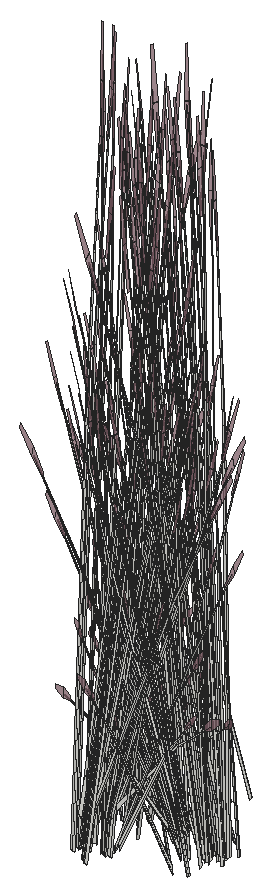
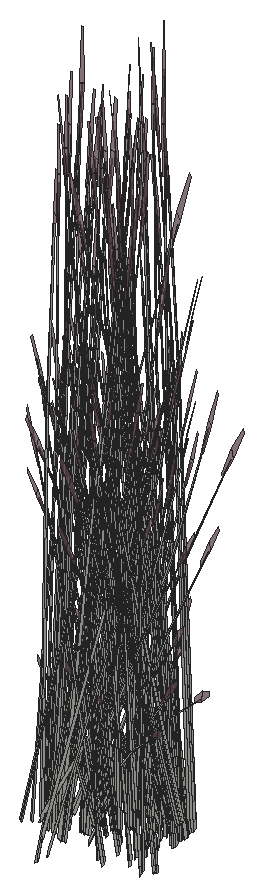
# SketchUp Ruby script. Lengths in inches.
U = 1.inch
M = Sketchup.active_model
def pt(a) = Geom::Point3d.new(a.map { |v| v * U })
def face(e, loops, mat)
  f = e.add_face(loops[0].map { |a| pt(a) })
  loops[1..].each { |l| e.add_face(l.map { |a| pt(a) }).erase! }
  f.material = f.back_material = mat if mat
  f
end
# faces: each face lists its corners as indices into pts; further lists are holes
def faces(e, pts, list, mat = nil) = list.each { |f| face(e, (f[0].is_a?(Array) ? f : [f]).map { |l| l.map { |i| pts[i] } }, mat) }
# xy, xz, yz: faces in a plane at the given z, y or x. An outline is a flat list of corners, or four numbers for a rectangle; further outlines are holes
def ring(l) = l.size == 4 ? [[l[0], l[1]], [l[2], l[1]], [l[2], l[3]], [l[0], l[3]]] : l.each_slice(2).to_a
def flat(e, list, mat, &to3) = list.each { |f| face(e, (f[0].is_a?(Array) ? f : [f]).map { |l| ring(l).map { |u, v| to3.(u, v) } }, mat) }
def xy(e, z, list, mat = nil) = flat(e, list, mat) { |x, y| [x, y, z] }
def xz(e, y, list, mat = nil) = flat(e, list, mat) { |x, z| [x, y, z] }
def yz(e, x, list, mat = nil) = flat(e, list, mat) { |y, z| [x, y, z] }
def lines(e, pts, list) = list.each { |a, b| e.add_line(pt(pts[a]), pt(pts[b])) }
# prism: a flat outline (further loops are holes) pulled along v
def prism(e, loops, v, mat = nil)
  f = face(e, loops, mat); d = Geom::Vector3d.new(v.map { |x| x * U })
  f.pushpull(f.normal.samedirection?(d) ? d.length : -d.length)
end
def box(e, o, s, mat = nil) = prism(e, [[o, [o[0] + s[0], o[1], o[2]], [o[0] + s[0], o[1] + s[1], o[2]], [o[0], o[1] + s[1], o[2]]]], [0, 0, s[2]], mat)
def at(x, y, z, deg = 0) = Geom::Transformation.translation(pt([x, y, z])) * Geom::Transformation.rotation(ORIGIN, Z_AXIS, deg.degrees)
def axes(o, x, y, z) = Geom::Transformation.new([*x, 0, *y, 0, *z, 0, *pt(o).to_a, 1])
def part(name) = M.definitions.add(name)
# library, detail: a bought-in or finely detailed component or shape, given as its bounding box
def library(name, o, s) = part(name).tap { |d| box(d.entities, o, s) }
def detail(e, o, s) = box(e.add_group.entities, o, s)
def put(e, d, t, mat = nil) = e.add_instance(d, t).tap { |i| i.material = mat if mat }
def group(e, t, mat = nil) = e.add_group.tap { |g| g.transformation = t; g.material = mat if mat }.entities
root = M.entities
M.materials.add("LightPink_Translucent").color = [144, 107, 117]
M.materials["LightPink_Translucent"].alpha = 0.75
c1 = part("blade")
p = [[2.15,0.21,22],[0,0.17,0],[0.09,0.45,0],[2.18,0.31,22],[2.29,0.31,22],[0.38,0.45,0],
  [2.48,0.24,33],[2.49,0.24,33],[2.48,0.22,33]]
faces(c1.entities,p,[[0,1,2,3],[4,5,2,3],[6,3,4,7],[8,0,3,6]])
c2 = part("seeds")
p = [[0.3,-0.1,1.38],[-0.01,-0.03,1.59],[-0.01,-0.03,0.03],[0.14,-0.07,-0.07],[0.29,-0.03,3],[0.15,0.01,3.11]]
faces(c2.entities,p,[[0,1,2,3],[1,0,4,5]],"LightPink_Translucent")
c3 = part("blade with seeds")
put(c3.entities,c1,at(0,0,0))
put(c3.entities,c2,axes([2.4,0.25,30.99],[1.5799,-0.05474,1.17369],[-0.12525,1.92788,0.29478],[-0.07173,-0.02425,1.56792]))
put(root,c3,axes([315.02,25.22,44.4],[-0.30332,-0.32798,0.39531],[0.45944,-0.23096,-0.19025],[0.09816,0.04058,1.26923]))
put(root,c3,axes([315.18,25.25,44.36],[0.50979,-0.25942,-0.25709],[0.339,0.36656,-0.44182],[0.12578,0.03723,1.41118]))
put(root,c3,axes([317.2,25.93,46],[0.41962,0.10901,-0.31292],[-0.12239,0.31802,0.40398],[0.16894,-0.02916,0.77298]))
put(root,c3,axes([321.92,27.46,46.18],[0.22948,-0.24822,0.05682],[0.32679,0.14452,0.44729],[-0.10565,-0.07958,0.68204]))
put(root,c3,axes([321.03,27.43,43.32],[-0.04891,0.05148,1.55816],[-0.49427,0.11098,-0.23804],[-0.1194,-0.10096,0.26541]))
put(root,c3,axes([316.46,24.56,43.78],[0.47255,0.19538,-0.43871],[-0.28245,0.35034,0],[0.10763,0.0445,1.3917]))
put(root,c3,axes([315.5625,25.67,43.95],[0.56491,0,0],[0,0.40454,0],[0,0,1.5764]))
put(root,c3,axes([321.85,28.84,43.85],[-0.20736,-0.4007,-0.61707],[0.59731,-0.14431,-0.16195],[-0.02292,-0.13569,1.36206]))
put(root,c3,axes([320.77,27.95,45.43],[0.18755,0.06732,1.51428],[-0.38813,0.28243,0.12244],[-0.24191,-0.12741,0.64734]))
put(root,c3,axes([315.72,24.72,44.1875],[-0.54257,0.10371,0.15589],[-0.13397,-0.38597,0.31002],[0.04839,0.05624,1.41735]))
put(root,c3,axes([316.06,25.54,45.43],[-0.20943,0.00885,1.51428],[0.13893,-0.38357,0.12244],[0.29846,0.02372,0.64734]))
put(root,c3,axes([323.06,27.7,46.46],[-0.15222,0.30049,0.31292],[-0.44409,-0.08764,-0.40398],[-0.04072,-0.12098,0.77298]))
put(root,c3,axes([316.33,24.7,43.79],[0.11861,0.34048,-0.27372],[-0.47106,0.09668,0.27372],[0.09497,0.03926,1.22797]))
put(root,c3,axes([321.67,27.75,46.14],[-0.49824,0.09289,-0.45151],[-0.08716,-0.35177,-0.34973],[-0.13382,-0.10081,0.86392]))
put(root,c3,axes([317.14,26.0625,46.18],[0.18545,0.26643,0.05682],[-0.33817,0.13041,0.44729],[0.14907,-0.02573,0.68204]))
put(root,c3,axes([322.02,27.43,46.8],[-0.33698,0.3746,-0.12034],[-0.48801,-0.21581,-0.66795],[-0.16964,-0.10584,1.01494]))
put(root,c3,axes([315.38,25.46,44.1],[-0.63817,-0.08233,0.43472],[0.12987,-0.46497,0.17059],[0.09326,0.0449,1.50931]))
put(root,c3,axes([317.11,25.97,46.18],[-0.14265,0.35629,0.42415],[-0.46898,-0.12183,0.34973],[0.18443,-0.02141,0.87768]))
put(root,c3,axes([315.49,26.57,43.93],[0.53009,-0.13258,-0.16963],[0.18627,0.38191,0.00007],[0.05851,-0.01465,1.53656]))
put(root,c3,axes([322.46,27.22,43.88],[-0.34892,0.22417,-0.0344],[-0.3197,-0.24551,-0.15595],[-0.02251,-0.06957,0.51438]))
put(root,c3,axes([315.55,25.84,43.96],[0.35245,0.2524,0],[-0.35245,0.2524,0],[0,0,1.49564]))
put(root,c3,axes([315.77,25.3,43.82],[0.52523,0.06406,-0.55095],[-0.11084,0.39517,-0.1446],[0.15674,0.04788,1.21613]))
put(root,c3,axes([320.73,27.33,46.17],[-0.10864,-0.00276,1.54581],[-0.34587,0.27582,-0.24447],[-0.18454,-0.05636,0.12397]))
put(root,c3,axes([318.09,25.99,44.44],[-0.31197,0.06451,1.01491],[0.14684,-0.26661,0.74569],[0.1655,0.01824,0.22354]))
put(root,c3,axes([315.6875,29.41,44.29],[-0.14352,0.07909,1.26356],[-0.42983,-0.13843,-0.27174],[0.07968,-0.17216,0.54024]))
put(root,c3,axes([322.91,29.875,44.9375],[0.43633,0.15757,1.33654],[-0.42745,0.33945,0.52853],[-0.19146,-0.20119,1.12046]))
put(root,c3,axes([315.55,25.55,44.4],[0.24498,-0.3521,0.39531],[0.50902,0.16945,-0.19025],[0,0.08116,1.26923]))
put(root,c3,axes([317.95,27.12,46.16],[-0.04566,-0.03421,1.56736],[0.09987,-0.36669,-0.1481],[0.17984,-0.02343,0.27737]))
put(root,c3,axes([321.99,27.75,46.46],[0.07798,0.31474,0.31292],[-0.44579,0.08311,-0.40398],[-0.11974,-0.09019,0.77298]))
put(root,c3,axes([320.625,28.79,43.78],[0,-0.39075,-0.43871],[0.56491,0,0],[0,-0.089,1.3917]))
put(root,c3,axes([320.65,27.95,46.5],[0.41698,-0.28837,0.47505],[0.35962,0.30624,0.3917],[-0.19563,-0.05319,0.983]))
put(root,c3,axes([315.5,25.43,43.95],[0.30332,0.32798,-0.39531],[-0.45944,0.23096,0.19025],[0.09816,0.04058,1.26923]))
put(root,c3,axes([317.55,26.82,45.47],[-0.09664,-0.32847,-0.03085],[0.45676,-0.07551,-0.13989],[0.09538,0.02082,0.4614]))
put(root,c3,axes([316.04,29.99,46.4],[0.01314,-0.36145,-0.62776],[0.55324,0.02428,0.07576],[0.05838,-0.15313,0.88802]))
put(root,c3,axes([316.37,26.81,46.45],[0.02704,-0.39739,-0.10745],[0.51189,0.01086,-0.59638],[0.19715,0.0276,0.90619]))
put(root,c3,axes([316.83,25.75,44.19],[0,-0.39075,0.43871],[0.56491,0,0],[0,0.089,1.3917]))
put(root,c3,axes([316.81,29.43,46.17],[-0.00487,-0.07777,1.54581],[-0.41166,-0.22476,-0.24447],[0.06364,-0.13625,0.12397]))
put(root,c3,axes([315.41,29.8125,45.43],[-0.09401,0.13431,1.51428],[-0.3944,-0.27795,0.12244],[0.17792,-0.17323,0.64734]))
put(root,c3,axes([316.7,29.15,46.16],[-0.05128,0.02985,1.56736],[-0.5024,-0.1007,-0.1481],[-0.01819,-0.13025,0.27737]))
put(root,c3,axes([315.76,25.63,44.3125],[0.47043,-0.11396,0.12794],[0.16474,0.32541,-0.36534],[0,0.07162,1.11991]))
put(root,c3,axes([316.29,26.65,46.46],[-0.28729,-0.24465,0.31292],[0.32804,-0.23159,-0.40398],[0.16667,0.03524,0.77298]))
put(root,c3,axes([320.84,27.95,46.18],[0.02542,-0.29714,0.05682],[0.38391,0.00815,0.44729],[-0.14706,-0.03109,0.68204]))
put(root,c3,axes([315.16,28.78,44.44],[0.06477,0.22786,1.01491],[-0.35932,-0.1262,0.74569],[0.03867,-0.11667,0.22354]))
put(root,c3,axes([317.51,26.42,44.29],[-0.1216,-0.0961,1.26356],[0.15822,-0.31792,-0.27174],[0.24603,0.04307,0.54024]))
put(root,c3,axes([322.16,28.95,43.95],[0.24498,-0.3521,-0.39531],[0.50902,0.16945,0.19025],[0,-0.08116,1.26923]))
put(root,c3,axes([320.69,28.04,46],[-0.28729,-0.24465,-0.31292],[0.32804,-0.23159,0.40398],[-0.16667,-0.03524,0.77298]))
put(root,c3,axes([315.92,29.875,46.14],[-0.36145,-0.26255,-0.45151],[0.38183,-0.22994,-0.34973],[0.055,-0.1334,0.86392]))
put(root,c3,axes([320.87,28.79,43.79],[0.35245,-0.2438,-0.27372],[0.35245,0.2438,0.27372],[0,-0.07853,1.22797]))
put(root,c3,axes([315.33,26.77,43.95],[0.50902,0.17543,0],[-0.24498,0.36452,0],[0,0,1.54589]))
put(root,c3,axes([320.72,27.625,43.88],[-0.14565,0.31907,-0.0344],[-0.44829,-0.09815,-0.15595],[-0.06806,-0.05219,0.51438]))
put(root,c3,axes([322.1,29.24,44.36],[-0.56863,-0.18645,-0.25709],[0.2738,-0.39352,-0.44182],[-0.01787,-0.09662,1.41118]))
put(root,c3,axes([320.48,29.08,44.1],[-0.63136,0,0],[0,-0.43672,-0.456],[0,-0.09947,1.44655]))
put(root,c3,axes([316.8125,26.57,46.17],[0.10831,-0.00661,1.54581],[0.29709,-0.30358,-0.24447],[0.19266,0.04007,0.12397]))
put(root,c3,axes([320.59,28.3,44.29],[0.09858,0.10879,1.26356],[-0.22716,0.29571,-0.27174],[-0.23325,-0.07068,0.54024]))
put(root,c3,axes([316.3,30.01,46.45],[-0.55492,-0.01936,-0.10745],[0.01517,-0.36657,-0.59638],[0.03855,-0.14118,0.90619]))
put(root,c3,axes([321,28.21,46.4],[-0.50473,-0.00941,-0.62776],[0.0339,-0.39618,0.07576],[-0.21383,-0.04181,0.88802]))
put(root,c3,axes([316.26,29.78,46],[0.34164,-0.20573,-0.31292],[0.3234,0.23491,0.40398],[0.04921,-0.11936,0.77298]))
put(root,c3,axes([316.39,26.62,46.4],[0.50473,0.00941,-0.62776],[-0.0339,0.39618,0.07576],[0.21383,0.04181,0.88802]))
put(root,c3,axes([320.97,28.97,44.06],[-0.46965,0.32852,0.27176],[-0.46994,-0.32506,-0.32244],[-0.0164,-0.09329,1.45692]))
put(root,c3,axes([317.22,25.8125,44.1],[0.63136,0,0],[0,0.43672,-0.456],[0,0.09947,1.44655]))
put(root,c3,axes([320.3125,27.56,46.16],[0.03743,0.039,1.56736],[-0.18045,0.35054,-0.1481],[-0.18276,0.00254,0.27737]))
put(root,c3,axes([315.6,25.66,44.36],[0.56863,0.18645,-0.25709],[-0.2738,0.39352,-0.44182],[0.01787,0.09662,1.41118]))
put(root,c3,axes([316.7,26.78,46],[0.28729,0.24465,-0.31292],[-0.32804,0.23159,0.40398],[0.16667,0.03524,0.77298]))
put(root,c3,axes([316.83,26.1,43.79],[-0.35245,0.2438,-0.27372],[-0.35245,-0.2438,0.27372],[0,0.07853,1.22797]))
put(root,c3,axes([322.24,29.65,44.16],[0.13383,-0.46302,-0.20702],[0.63453,0.08071,0.45303],[-0.11087,-0.06394,1.38231]))
put(root,c3,axes([316.6875,29.65,43.32],[-0.07557,-0.03078,1.55816],[-0.19412,-0.34391,-0.23804],[0.13095,-0.09333,0.26541]))
put(root,c3,axes([316.55,26.87,46.18],[-0.02542,0.29714,0.05682],[-0.38391,-0.00815,0.44729],[0.14706,0.03109,0.68204]))
put(root,c3,axes([320.83,28.29,46.14],[-0.36663,0.25884,-0.45151],[-0.32109,-0.27343,-0.34973],[-0.18628,-0.03938,0.86392]))
put(root,c3,axes([321.1,28.17,46.46],[0.28729,0.24465,0.31292],[-0.32804,0.23159,-0.40398],[-0.16667,-0.03524,0.77298]))
put(root,c3,axes([316.58,26.78,46.18],[-0.3723,0.25748,0.42415],[-0.32109,-0.27343,0.34973],[0.17467,0.04749,0.87768]))
put(root,c3,axes([320,28.63,44.44],[0.32236,-0.02796,1.01491],[-0.20448,0.24636,0.74569],[-0.1593,-0.03696,0.22354]))
put(root,c3,axes([316.26,29.86,46.18],[0.35954,0.26661,0.42415],[-0.38183,0.22994,0.34973],[0.06632,-0.12508,0.87768]))
put(root,c3,axes([316.39,29.88,46.18],[0.41493,0.01821,0.05682],[-0.01138,0.27493,0.44729],[0.04342,-0.10531,0.68204]))
put(root,c3,axes([321.02,28.01,46.45],[-0.02704,0.39739,-0.10745],[-0.51189,-0.01086,-0.59638],[-0.19715,-0.0276,0.90619]))
put(root,c3,axes([320.87,29.15,44.19],[0,0.39075,0.43871],[-0.56491,0,0],[0,-0.089,1.3917]))
put(root,c3,axes([316.08,30.07,46.46],[-0.34164,0.20573,0.31292],[-0.3234,-0.23491,-0.40398],[0.04921,-0.11936,0.77298]))
put(root,c3,axes([316.6875,30.62,46.4],[0.26374,-0.30832,-0.62776],[0.46217,0.21911,0.07576],[0.15748,-0.11171,0.88802]))
put(root,c3,axes([322.2,29.46,43.95],[-0.30332,-0.32798,-0.39531],[0.45944,-0.23096,0.19025],[-0.09816,-0.04058,1.26923]))
put(root,c3,axes([322.26,29,44.09],[0.21952,0.43694,0.40429],[-0.62724,0.15194,0.15865],[0.00767,-0.08029,1.40366]))
put(root,c3,axes([316.67,30.48,46.14],[-0.12971,-0.3568,-0.45151],[0.49122,-0.06241,-0.34973],[0.14077,-0.09583,0.86392]))
put(root,c3,axes([315.4,27.08,46.46],[-0.07798,-0.31474,0.31292],[0.44579,-0.08311,-0.40398],[0.11974,0.09019,0.77298]))
put(root,c3,axes([317.08,26.11,43.78],[0,0.39075,-0.43871],[-0.56491,0,0],[0,0.089,1.3917]))
put(root,c3,axes([315.66,26.15,45.43],[-0.18755,-0.06732,1.51428],[0.38813,-0.28243,0.12244],[0.24191,0.12741,0.64734]))
put(root,c3,axes([322.15,29.34,44.4],[-0.24498,0.3521,0.39531],[-0.50902,-0.16945,-0.19025],[0,-0.08116,1.26923]))
put(root,c3,axes([315.7,25.27,45.95],[-0.4363,-0.20303,1.22187],[0.46069,-0.31611,0.5272],[0.14077,0.1905,1.18105]))
put(root,c3,axes([316.91,30.73,46.45],[-0.46706,-0.21546,-0.10745],[0.26908,-0.31203,-0.59638],[0.13196,-0.10846,0.90619]))
put(root,c3,axes([316.36,26.92,44.44],[-0.28429,-0.11236,1.01491],[0.36709,-0.11416,0.74569],[0.09901,0.0967,0.22354]))
put(root,c3,axes([315.36,27.24,46.45],[0.30087,-0.33447,-0.10745],[0.43572,0.19269,-0.59638],[0.15146,0.0945,0.90619]))
put(root,c3,axes([321.93,29.59,43.82],[-0.52523,-0.06406,-0.55095],[0.11084,-0.39517,-0.1446],[-0.15674,-0.04788,1.21613]))
put(root,c3,axes([323.21,29.39,44.03],[-0.46965,-0.33633,-0.05417],[0.46994,-0.33653,0],[-0.0164,-0.01174,1.55135]))
put(root,c3,axes([314.26,29.66,43.78],[0.47255,-0.19538,-0.43871],[0.28245,0.35034,0],[0.10763,-0.0445,1.3917]))
put(root,c3,axes([317.07,30.34,44.29],[-0.18038,-0.01157,1.26356],[-0.18479,-0.31048,-0.27174],[0.22159,-0.08783,0.54024]))
put(root,c3,axes([318.06,30.64,46.16],[-0.06595,-0.00297,1.56736],[-0.27386,-0.31799,-0.1481],[0.10998,-0.10455,0.27737]))
put(root,c3,axes([320.29,28.85,46.18],[0.14265,-0.35629,0.42415],[0.46898,0.12183,0.34973],[-0.18443,0.02141,0.87768]))
put(root,c3,axes([314.97,27.52,46.16],[0.00149,-0.04731,1.56736],[0.4327,-0.20872,-0.1481],[0.1503,0.0745,0.27737]))
put(root,c3,axes([314.82,30.47,43.82],[0.34009,-0.2937,-0.55095],[0.42248,0.26632,-0.1446],[0.13628,-0.07327,1.21613]))
put(root,c3,axes([316.4375,27.34,43.32],[0.03679,-0.05641,1.55816],[0.46313,-0.16615,-0.23804],[0.14041,0.08599,0.26541]))
put(root,c3,axes([317.28,29.77,44.44],[-0.16818,0.19891,1.01491],[-0.14456,-0.26725,0.74569],[0.1389,-0.06697,0.22354]))
put(root,c3,axes([315.83,26.05,43.85],[0.18514,0.35777,-0.61156],[-0.53331,0.12885,-0.16051],[0.02046,0.12115,1.3499]))
put(root,c3,axes([320.25,28.76,46.18],[-0.18545,-0.26643,0.05682],[0.33817,-0.13041,0.44729],[-0.14907,0.02573,0.68204]))
put(root,c3,axes([322.32,29.43,44.09],[0.63817,0.08233,0.40429],[-0.12987,0.46497,0.15865],[-0.09326,-0.0449,1.40366]))
put(root,c3,axes([315.72,27.07,46.14],[0.49824,-0.09289,-0.45151],[0.08716,0.35177,-0.34973],[0.13382,0.10081,0.86392]))
put(root,c3,axes([320.24,29.03,43.32],[0.0128,0.06158,1.55816],[-0.25814,0.3216,-0.23804],[-0.18336,-0.01621,0.26541]))
put(root,c3,axes([317.04,30.52,46],[0.43951,-0.05584,-0.31292],[0.11606,0.31924,0.40398],[0.12595,-0.08575,0.77298]))
put(root,c3,axes([321.37,30.19,43.79],[-0.11861,-0.34048,-0.27372],[0.47106,-0.09668,0.27372],[-0.09497,-0.03926,1.22797]))
put(root,c3,axes([316.4,27.43,44.36],[-0.32378,-0.01225,0.92831],[0.21383,-0.26028,0.51254],[0.12791,0.09247,0.72818]))
put(root,c3,axes([314.46,30.81,44.36],[-0.05884,-0.44587,-0.25709],[0.6128,-0.02696,-0.44182],[0.10791,-0.05939,1.41118]))
put(root,c3,axes([321.98,30.17,44.1875],[0.54257,-0.10371,0.15589],[0.13397,0.38597,0.31002],[-0.04839,-0.05624,1.41735]))
put(root,c3,axes([315.47,27.36,46.18],[-0.22948,0.24822,0.05682],[-0.32679,-0.14452,0.44729],[0.10565,0.07958,0.68204]))
put(root,c3,axes([316.68,30.7,46.46],[-0.43951,0.05584,0.31292],[-0.11606,-0.31924,-0.40398],[0.12595,-0.08575,0.77298]))
put(root,c3,axes([321.24,30.34,43.78],[-0.47255,-0.19538,-0.43871],[0.28245,-0.35034,0],[-0.10763,-0.0445,1.3917]))
put(root,c3,axes([314.93,28.2,46.99],[0.34892,-0.22417,-0.05733],[0.3197,0.24551,-0.25992],[0.02251,0.06957,0.85731]))
put(root,c3,axes([320.1875,28.89,46],[-0.41962,-0.10901,-0.31292],[0.12239,-0.31802,0.40398],[-0.16894,0.02916,0.77298]))
put(root,c3,axes([315.57,27.29,46.18],[-0.5022,0.08967,0.42415],[-0.08716,-0.35177,0.34973],[0.11811,0.10367,0.87768]))
put(root,c3,axes([322.52,29.65,44.36],[-0.50979,0.25942,-0.25709],[-0.339,-0.36656,-0.44182],[-0.12578,-0.03723,1.41118]))
put(root,c3,axes([314.375,29.82,43.79],[0.47106,0.09668,-0.27372],[-0.11861,0.34048,0.27372],[0.09497,-0.03926,1.22797]))
put(root,c3,axes([315.35,26.8,44.29],[0.00891,-0.12953,1.26356],[0.4258,-0.14469,-0.27174],[0.13144,0.15503,0.54024]))
put(root,c3,axes([314.18,27.25,46.45],[0.49409,-0.18193,-0.10745],[0.24281,0.32289,-0.59638],[0.06519,0.13607,0.90619]))
put(root,c3,axes([317.08,30.65,46.18],[0.34663,0.16434,0.05682],[-0.20181,0.23402,0.44729],[0.11113,-0.07566,0.68204]))
put(root,c3,axes([322.79,30.08,43.95],[-0.16474,-0.33688,0],[0.47043,-0.11798,0],[0,0,1.36402]))
put(root,c3,axes([316.98,30.58,46.18],[0.12522,0.35963,0.42415],[-0.49122,0.06241,0.34973],[0.14477,-0.08458,0.87768]))
put(root,c3,axes([322.48,29.76,44.3125],[-0.09741,0.34873,0.12794],[-0.4759,-0.06053,-0.36534],[-0.08661,-0.03581,1.11991]))
put(root,c3,axes([318.3,31.02,46.17],[0.07006,-0.05952,1.54581],[-0.08968,-0.3651,-0.24447],[0.1758,-0.06922,0.12397]))
put(root,c3,axes([320.63,28.86,46.46],[0.41962,0.10901,0.31292],[-0.12239,0.31802,-0.40398],[-0.16894,0.02916,0.77298]))
put(root,c3,axes([323.59,30.19,44.1875],[0.14586,-0.38834,0.15589],[0.53375,0.1099,0.31002],[-0.0922,0.00189,1.41735]))
put(root,c3,axes([321.47,28.84,44.95],[0.14352,-0.05653,1.56454],[0.04949,0.39467,0.12244],[-0.31087,0.05237,0.55918]))
put(root,c3,axes([314.61,27.24,46.14],[0.49634,0.09796,-0.45151],[-0.17013,0.33585,-0.34973],[0.04551,0.13522,0.86392]))
put(root,c3,axes([322.67,30.23,43.94],[-0.50902,-0.17543,0],[0.24498,-0.36452,0],[0,0,1.43768]))
put(root,c3,axes([323.1,29.77,44.18],[-0.49304,-0.31451,-0.2226],[0.41487,-0.35316,0.48713],[-0.13277,0.03679,1.48635]))
put(root,c3,axes([314.89,26.54,45.43],[-0.11542,-0.12546,1.51428],[0.53333,-0.10562,0.12244],[0.12054,0.19696,0.64734]))
put(root,c3,axes([321.8,30.37,44.19],[0.47255,0.19538,0.43871],[-0.28245,0.35034,0],[-0.10763,-0.0445,1.3917]))
put(root,c3,axes([320.52,33.41,45.43],[0.11542,0.12546,1.51428],[-0.53333,0.10562,0.12244],[-0.12054,-0.19696,0.64734]))
put(root,c3,axes([319.92,29.1,46.17],[-0.08245,0.05073,1.54581],[0.00701,0.37067,-0.24447],[-0.18899,0.0482,0.12397]))
put(root,c3,axes([320.48,29.05,46.14],[-0.13679,0.35544,-0.45151],[-0.46898,-0.12183,-0.34973],[-0.18882,0.03259,0.86392]))
put(root,c3,axes([321.4,32.58,46.17],[-0.07723,-0.05479,1.54581],[-0.51538,0.03473,-0.24447],[-0.08225,-0.13104,0.12397]))
put(root,c3,axes([320.45,28.75,46.45],[0.25405,0.35383,-0.10745],[-0.45089,0.17388,-0.59638],[-0.19001,0.04668,0.90619]))
put(root,c3,axes([316.92,31.57,46.45],[-0.25405,-0.35383,-0.10745],[0.45089,-0.17388,-0.59638],[0.19001,-0.04668,0.90619]))
put(root,c3,axes([321.53,30.57,44.1],[-0.31568,0.39156,0],[-0.52815,-0.21836,-0.456],[-0.12029,-0.04973,1.44655]))
put(root,c3,axes([316.9,31.27,46.14],[0.13679,-0.35544,-0.45151],[0.46898,0.12183,-0.34973],[0.18882,-0.03259,0.86392]))
put(root,c3,axes([316.16,29.82,44.1],[0.31568,-0.39156,0],[0.52815,0.21836,-0.456],[0.12029,0.04973,1.44655]))
put(root,c3,axes([321.94,33.51,46.4],[-0.24099,-0.31773,-0.62776],[0.49607,-0.17707,0.07576],[-0.05635,-0.15352,0.88802]))
put(root,c3,axes([323.34,29.51,44.4],[0.54829,-0.02412,0.39531],[0.04958,0.40041,-0.19025],[-0.09816,0.04058,1.26923]))
put(root,c3,axes([320.375,33.08,44.29],[-0.03058,0.12783,1.26356],[-0.44698,0.10701,-0.27174],[-0.10448,-0.16522,0.54024]))
put(root,c3,axes([317.4,31.37,43.75],[-0.3252,0.04689,1.25103],[-0.05176,-0.37326,0.07161],[0.22777,-0.0565,0.71188]))
put(root,c3,axes([318,31.04,44],[-0.31304,-0.24986,-0.05733],[0.34284,-0.22894,-0.25992],[0.09714,-0.01612,0.85731]))
put(root,c3,axes([322.85,29.7,43.95],[-0.54829,0.02412,-0.39531],[-0.04958,-0.40041,0.19025],[-0.09816,0.04058,1.26923]))
put(root,c3,axes([321.53,32.8,43.32],[-0.08469,0.01408,1.55816],[-0.46834,-0.15847,-0.23804],[0.00786,-0.13218,0.26541]))
put(root,c3,axes([315.89,30.03,44.19],[-0.47255,-0.19538,0.43871],[0.28245,-0.35034,0],[0.10763,0.0445,1.3917]))
